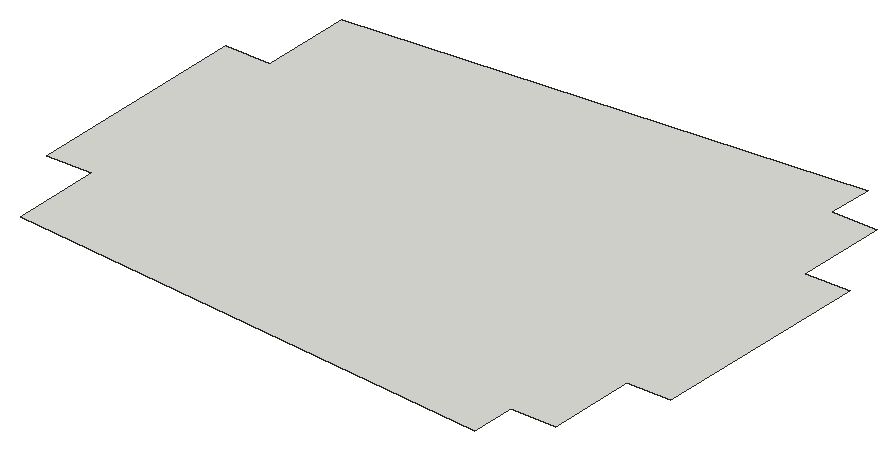
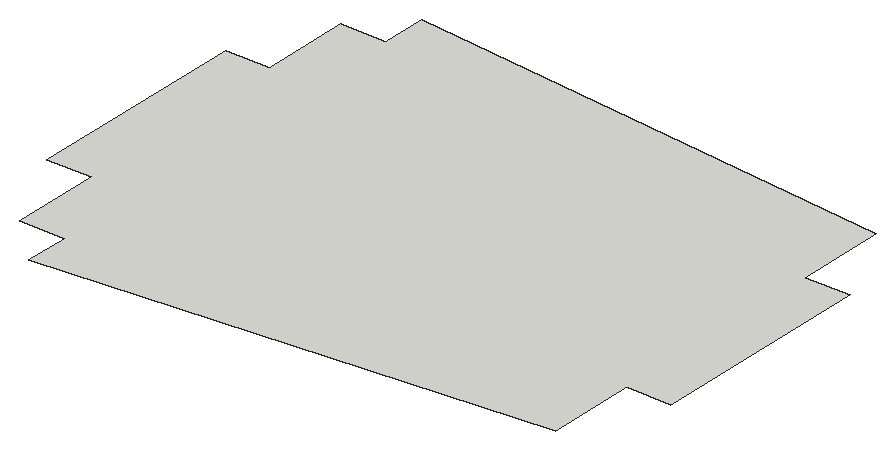
# SketchUp Ruby script. Lengths in inches.
U = 1.inch
M = Sketchup.active_model
def pt(a) = Geom::Point3d.new(a.map { |v| v * U })
def face(e, loops, mat)
  f = e.add_face(loops[0].map { |a| pt(a) })
  loops[1..].each { |l| e.add_face(l.map { |a| pt(a) }).erase! }
  f.material = f.back_material = mat if mat
  f
end
# faces: each face lists its corners as indices into pts; further lists are holes
def faces(e, pts, list, mat = nil) = list.each { |f| face(e, (f[0].is_a?(Array) ? f : [f]).map { |l| l.map { |i| pts[i] } }, mat) }
# xy, xz, yz: faces in a plane at the given z, y or x. An outline is a flat list of corners, or four numbers for a rectangle; further outlines are holes
def ring(l) = l.size == 4 ? [[l[0], l[1]], [l[2], l[1]], [l[2], l[3]], [l[0], l[3]]] : l.each_slice(2).to_a
def flat(e, list, mat, &to3) = list.each { |f| face(e, (f[0].is_a?(Array) ? f : [f]).map { |l| ring(l).map { |u, v| to3.(u, v) } }, mat) }
def xy(e, z, list, mat = nil) = flat(e, list, mat) { |x, y| [x, y, z] }
def xz(e, y, list, mat = nil) = flat(e, list, mat) { |x, z| [x, y, z] }
def yz(e, x, list, mat = nil) = flat(e, list, mat) { |y, z| [x, y, z] }
def lines(e, pts, list) = list.each { |a, b| e.add_line(pt(pts[a]), pt(pts[b])) }
# prism: a flat outline (further loops are holes) pulled along v
def prism(e, loops, v, mat = nil)
  f = face(e, loops, mat); d = Geom::Vector3d.new(v.map { |x| x * U })
  f.pushpull(f.normal.samedirection?(d) ? d.length : -d.length)
end
def box(e, o, s, mat = nil) = prism(e, [[o, [o[0] + s[0], o[1], o[2]], [o[0] + s[0], o[1] + s[1], o[2]], [o[0], o[1] + s[1], o[2]]]], [0, 0, s[2]], mat)
def at(x, y, z, deg = 0) = Geom::Transformation.translation(pt([x, y, z])) * Geom::Transformation.rotation(ORIGIN, Z_AXIS, deg.degrees)
def axes(o, x, y, z) = Geom::Transformation.new([*x, 0, *y, 0, *z, 0, *pt(o).to_a, 1])
def part(name) = M.definitions.add(name)
# library, detail: a bought-in or finely detailed component or shape, given as its bounding box
def library(name, o, s) = part(name).tap { |d| box(d.entities, o, s) }
def detail(e, o, s) = box(e.add_group.entities, o, s)
def put(e, d, t, mat = nil) = e.add_instance(d, t).tap { |i| i.material = mat if mat }
def group(e, t, mat = nil) = e.add_group.tap { |g| g.transformation = t; g.material = mat if mat }.entities
root = M.entities
xy(root,0,[[16.251,358.886,16.27,358.886,16.274,358.887,16.279,358.888,16.283,358.889,16.287,358.891,16.292,358.893,16.297,358.896,16.301,358.899,16.306,358.903,16.31,358.906,16.313,358.91,16.317,358.915,16.32,358.919,16.323,358.924,16.325,358.929,16.326,358.933,16.328,358.9375,16.329,358.942,16.33,358.946,16.33,358.964,16.329,358.969,16.328,358.973,16.326,358.978,16.325,358.982,16.323,358.987,16.32,358.992,16.317,358.996,16.313,359.001,16.31,359.005,16.306,359.008,16.301,359.012,16.297,359.015,16.292,359.017,16.287,359.02,16.283,359.021,16.279,359.023,16.274,359.024,16.27,359.024,16.265,359.025,16.256,359.025,16.251,359.024,16.247,359.024,16.243,359.023,16.238,359.021,16.234,359.02,16.229,359.017,16.224,359.015,16.22,359.012,16.215,359.008,16.211,359.005,16.208,359.001,16.204,358.996,16.201,358.992,16.199,358.987,16.196,358.982,16.195,358.978,16.193,358.973,16.192,358.969,16.192,358.964,16.191,358.96,16.191,358.951,16.192,358.946,16.192,358.942,16.193,358.9375,16.195,358.933,16.196,358.929,16.199,358.924,16.201,358.919,16.204,358.915,16.208,358.91,16.211,358.906,16.215,358.903,16.22,358.899,16.224,358.896,16.229,358.893,16.234,358.891,16.238,358.889,16.243,358.888]])
